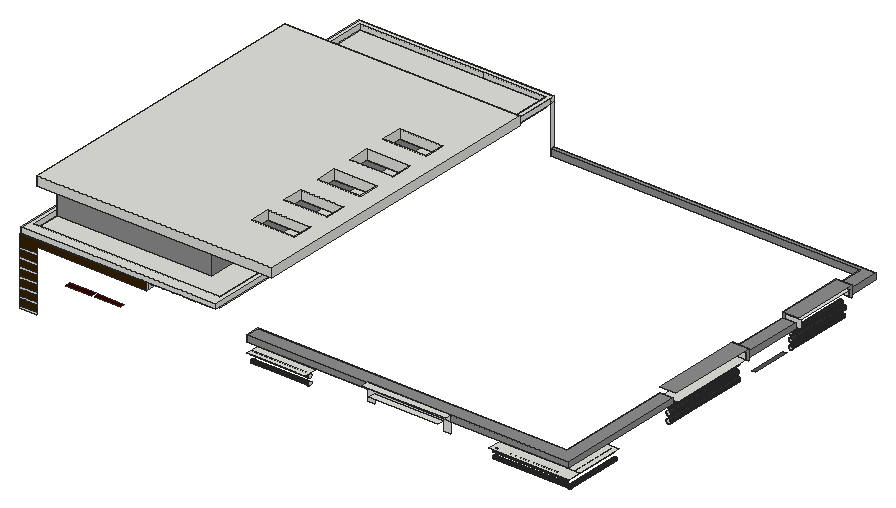
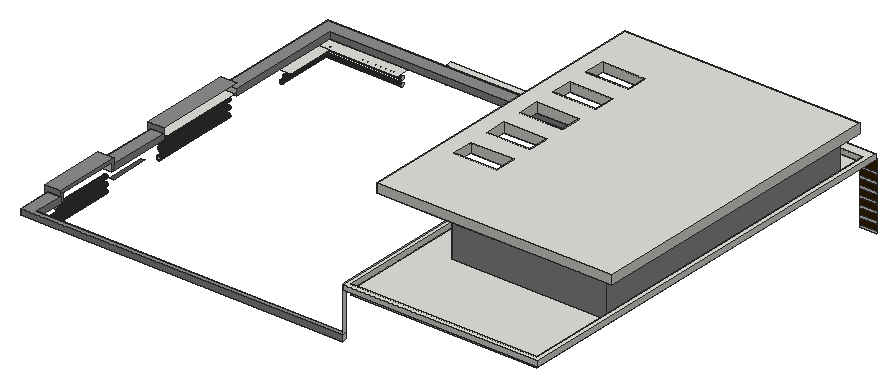
# SketchUp Ruby script. Lengths in inches.
U = 1.inch
M = Sketchup.active_model
def pt(a) = Geom::Point3d.new(a.map { |v| v * U })
def face(e, loops, mat)
  f = e.add_face(loops[0].map { |a| pt(a) })
  loops[1..].each { |l| e.add_face(l.map { |a| pt(a) }).erase! }
  f.material = f.back_material = mat if mat
  f
end
# faces: each face lists its corners as indices into pts; further lists are holes
def faces(e, pts, list, mat = nil) = list.each { |f| face(e, (f[0].is_a?(Array) ? f : [f]).map { |l| l.map { |i| pts[i] } }, mat) }
# xy, xz, yz: faces in a plane at the given z, y or x. An outline is a flat list of corners, or four numbers for a rectangle; further outlines are holes
def ring(l) = l.size == 4 ? [[l[0], l[1]], [l[2], l[1]], [l[2], l[3]], [l[0], l[3]]] : l.each_slice(2).to_a
def flat(e, list, mat, &to3) = list.each { |f| face(e, (f[0].is_a?(Array) ? f : [f]).map { |l| ring(l).map { |u, v| to3.(u, v) } }, mat) }
def xy(e, z, list, mat = nil) = flat(e, list, mat) { |x, y| [x, y, z] }
def xz(e, y, list, mat = nil) = flat(e, list, mat) { |x, z| [x, y, z] }
def yz(e, x, list, mat = nil) = flat(e, list, mat) { |y, z| [x, y, z] }
def lines(e, pts, list) = list.each { |a, b| e.add_line(pt(pts[a]), pt(pts[b])) }
# prism: a flat outline (further loops are holes) pulled along v
def prism(e, loops, v, mat = nil)
  f = face(e, loops, mat); d = Geom::Vector3d.new(v.map { |x| x * U })
  f.pushpull(f.normal.samedirection?(d) ? d.length : -d.length)
end
def box(e, o, s, mat = nil) = prism(e, [[o, [o[0] + s[0], o[1], o[2]], [o[0] + s[0], o[1] + s[1], o[2]], [o[0], o[1] + s[1], o[2]]]], [0, 0, s[2]], mat)
def at(x, y, z, deg = 0) = Geom::Transformation.translation(pt([x, y, z])) * Geom::Transformation.rotation(ORIGIN, Z_AXIS, deg.degrees)
def axes(o, x, y, z) = Geom::Transformation.new([*x, 0, *y, 0, *z, 0, *pt(o).to_a, 1])
def part(name) = M.definitions.add(name)
# library, detail: a bought-in or finely detailed component or shape, given as its bounding box
def library(name, o, s) = part(name).tap { |d| box(d.entities, o, s) }
def detail(e, o, s) = box(e.add_group.entities, o, s)
def put(e, d, t, mat = nil) = e.add_instance(d, t).tap { |i| i.material = mat if mat }
def group(e, t, mat = nil) = e.add_group.tap { |g| g.transformation = t; g.material = mat if mat }.entities
root = M.entities
M.materials.add("[Color A08]").color = [56, 34, 0]
M.materials.add("[Color A08]1").color = [63, 0, 0]
M.materials.add("[Color M04]").color = [142, 142, 142]
M.materials.add("[Color M06]").color = [86, 86, 86]
M.materials.add("[Color M07]").color = [58, 58, 58]
xy(root,396,[[746.25,843.78,750.625,894.65]],"[Color M06]")
xy(root,403.48,[[329.75,539.27,405.75,557.27],[645.89,539.27,750.625,557.27],[733.6875,557.27,750.625,621.15]])
xy(root,415.22,[[496.66,529.59,587.54,539.27]])
xy(root,417,[[329.75,539.27,750.625,557.27],[733.6875,557.27,750.625,709.18],[733.6875,828.03,750.625,909.39],[733.6875,996.8,733.6875,1035.15,329.75,1035.15,329.75,1041.15,750.625,1041.15,750.625,996.8]])
xy(root,419.97,[[733.6875,712.4,754.75,823.78]])
xy(root,424.875,[[329.75,539.27,750.625,539.27,750.625,709.18,733.6875,709.18,733.6875,557.27,329.75,557.27],[733.6875,828.03,750.625,909.39],[733.6875,996.8,750.625,996.8,750.625,1041.15,329.75,1041.15,329.75,1035.15,733.6875,1035.15]],"[Color M04]")
xy(root,425.5625,[[488.01,529.59,597.14,539.27]])
xy(root,428.02,[[733.6875,912.34,754.75,992.73]])
xy(root,430.67,[[128.05,496.71,161.69,502.71],[165.04,496.71,198.99,502.71]],"[Color A08]1")
xy(root,431.5625,[[733.6875,709.18,754.75,828.03],[733.6875,909.39,754.75,996.8]],"[Color M04]")
xy(root,468.42,[[96.69,487.84,233.4,496.71],[233.4,487.84,241.19,496.71]])
xy(root,471,[[81.5,502.71,323.75,1035.15]])
xy(root,477,[[75.5,487.84,233.4,489.27],[233.4,487.84,241.19,489.27],[241.19,489.02,247.4,489.27],[255.19,489.02,261.4,489.27],[269.19,489.02,275.4,489.27],
  [283.19,489.02,289.4,489.27],[297.19,489.02,303.4,489.27],[75.5,489.27,233.4,496.71],[233.4,489.27,241.19,496.71],[241.19,489.27,247.4,496.71],
  [247.4,489.27,255.19,496.71],[255.19,489.27,261.4,496.71],[261.4,489.27,269.19,496.71],[269.19,489.27,275.4,496.71],[275.4,489.27,283.19,496.71],
  [283.19,489.27,289.4,496.71],[289.4,489.27,297.19,496.71],[297.19,489.27,303.4,496.71],[303.4,489.27,311.19,496.71],[311.19,489.27,317.4,496.71],
  [317.4,489.27,325.19,496.71],[81.5,502.71,323.75,502.71,323.75,1035.15,81.5,1035.15,81.5,920.84,283.1875,920.84,283.1875,540.53,81.5,540.53]])
xy(root,483.8125,[[[75.5,489.27,329.75,1041.15],[81.5,502.71,323.75,1035.15]]])
xy(root,519.8125,[[73.9375,516.34,81.5,920.84],[[81.5,516.34,81.5,540.53,283.1875,540.53,283.1875,920.84,381.1875,920.84,381.1875,516.34],[303.02,580.77,358.89,608.21],[303.02,634.08,358.89,661.52],[303.02,688.46,358.89,715.89],[303.02,741.58,358.89,769.02],[303.02,795.89,358.89,823.33]],[81.5,540.53,283.1875,920.84]])
xy(root,531.8125,[[[73.9375,516.34,381.1875,920.84],[303.02,795.89,358.89,823.33],[303.02,741.58,358.89,769.02],[303.02,688.46,358.89,715.89],[303.02,634.08,358.89,661.52],[303.02,580.77,358.89,608.21]]])
xz(root,487.84,[[75.5,389.53,96.69,392.83],[75.5,401.03,96.69,404.33],[75.5,412.53,96.69,415.83],[75.5,424.03,96.69,427.33],[75.5,435.53,96.69,438.83],
  [75.5,447.03,96.69,450.33],[75.5,458.53,96.69,461.83]])
xz(root,487.84,[[75.5,392.83,96.69,401.03],[75.5,404.33,96.69,412.53],[75.5,415.83,96.69,424.03],[75.5,427.33,96.69,435.53],[75.5,438.83,96.69,447.03],
  [75.5,450.33,96.69,458.53],[75.5,461.83,96.69,461.83,96.69,468.42,241.19,468.42,241.19,477,75.5,477]],"[Color A08]")
xz(root,489.27,[[75.5,477,329.75,483.8125]])
xz(root,502.71,[[81.5,471,303.1875,477],[303.1875,471,323.75,477],[81.5,477,241.19,483.8125],[241.19,477,303.1875,483.8125],[303.1875,477,323.75,483.8125]])
xz(root,516.34,[[73.9375,519.8125,381.1875,531.8125]])
xz(root,539.27,[[488.01,403.48,488.01,417,597.14,417,597.14,403.48,587.54,403.48,587.54,415.22,496.66,415.22,496.66,403.48],[488.01,417,597.14,424.875],[488.01,424.875,597.14,425.5625]])
xz(root,539.27,[[329.75,417,488.01,424.875],[597.14,417,750.625,424.875]],"[Color M04]")
xz(root,540.53,[[81.5,477,283.1875,519.8125]],"[Color M04]")
xz(root,557.27,[[329.75,417,733.6875,424.875]],"[Color M04]")
xz(root,580.77,[[303.02,519.8125,358.89,531.8125]])
xz(root,608.21,[[303.02,519.8125,358.89,531.8125]])
xz(root,634.08,[[303.02,519.8125,358.89,531.8125]])
xz(root,661.52,[[303.02,519.8125,358.89,531.8125]])
xz(root,688.46,[[303.02,519.8125,358.89,531.8125]])
xz(root,709.18,[[733.6875,417,750.625,424.875]])
xz(root,712.4,[[742.21,389.57,742.97,389.67,743.68,389.97,744.29,390.43,744.75,391.04,745.05,391.75,745.15,392.51,745.05,393.27,744.75,393.98,744.29,394.59,743.68,395.06,742.97,395.35,742.21,395.45,741.45,395.35,740.74,395.06,740.13,394.59,739.67,393.98,739.37,393.27,739.27,392.51,739.37,391.75,739.67,391.04,740.13,390.43,740.74,389.97,741.45,389.67],[742.21,399.14,742.97,399.24,743.68,399.53,744.29,400,744.75,400.61,745.05,401.3125,745.15,402.07,745.05,402.83,744.75,403.54,744.29,404.15,743.68,404.62,742.97,404.91,742.21,405.01,741.45,404.91,740.74,404.62,740.13,404.15,739.67,403.54,739.37,402.83,739.27,402.07,739.37,401.3125,739.67,400.61,740.13,400,740.74,399.53,741.45,399.24],[742.21,408.57,742.97,408.67,743.68,408.97,744.29,409.43,744.75,410.04,745.05,410.75,745.15,411.51,745.05,412.27,744.75,412.98,744.29,413.59,743.68,414.06,742.97,414.35,742.21,414.45,741.45,414.35,740.74,414.06,740.13,413.59,739.67,412.98,739.37,412.27,739.27,411.51,739.37,410.75,739.67,410.04,740.13,409.43,740.74,408.97,741.45,408.67]])
xz(root,715.89,[[303.02,519.8125,358.89,531.8125]])
xz(root,741.58,[[303.02,519.8125,358.89,531.8125]])
xz(root,769.02,[[303.02,519.8125,358.89,531.8125]])
xz(root,795.89,[[303.02,519.8125,358.89,531.8125]])
xz(root,823.33,[[303.02,519.8125,358.89,531.8125]])
xz(root,824.97,[[742.21,408.57,741.45,408.67,740.74,408.97,740.13,409.43,739.67,410.04,739.37,410.75,739.27,411.51,739.37,412.27,739.67,412.98,740.13,413.59,740.74,414.06,741.45,414.35,742.21,414.45,742.97,414.35,743.68,414.06,744.29,413.59,744.75,412.98,745.05,412.27,745.15,411.51,745.05,410.75,744.75,410.04,744.29,409.43,743.68,408.97,742.97,408.67]])
xz(root,825.78,[[742.21,389.57,741.45,389.67,740.74,389.97,740.13,390.43,739.67,391.04,739.37,391.75,739.27,392.51,739.37,393.27,739.67,393.98,740.13,394.59,740.74,395.06,741.45,395.35,742.21,395.45,742.97,395.35,743.68,395.06,744.29,394.59,744.75,393.98,745.05,393.27,745.15,392.51,745.05,391.75,744.75,391.04,744.29,390.43,743.68,389.97,742.97,389.67]])
xz(root,828.03,[[733.6875,417,750.625,424.875]])
xz(root,828.03,[[750.625,417,750.625,424.875,733.6875,424.875,733.6875,431.5625,754.75,431.5625,754.75,417]],"[Color M04]")
xz(root,909.39,[[733.6875,417,750.625,424.875]])
xz(root,912.34,[[741.96,388.71,742.64,388.8,743.28,389.06,743.82,389.48,744.24,390.02,744.5,390.65,744.59,391.33,744.5,392.01,744.24,392.65,743.82,393.1875,743.28,393.61,742.64,393.87,741.96,393.96,741.28,393.87,740.65,393.61,740.11,393.1875,739.69,392.65,739.43,392.01,739.34,391.33,739.43,390.65,739.69,390.02,740.11,389.48,740.65,389.06,741.28,388.8],[741.96,397.33,742.64,397.42,743.28,397.68,743.82,398.1,744.24,398.65,744.5,399.28,744.59,399.96,744.5,400.64,744.24,401.27,743.82,401.8125,743.28,402.23,742.64,402.49,741.96,402.58,741.28,402.49,740.65,402.23,740.11,401.8125,739.69,401.27,739.43,400.64,739.34,399.96,739.43,399.28,739.69,398.65,740.11,398.1,740.65,397.68,741.28,397.42],[741.96,406.27,742.64,406.36,743.28,406.62,743.82,407.04,744.24,407.58,744.5,408.22,744.59,408.9,744.5,409.57,744.24,410.21,743.82,410.75,743.28,411.17,742.64,411.43,741.96,411.52,741.28,411.43,740.65,411.17,740.11,410.75,739.69,410.21,739.43,409.57,739.34,408.9,739.43,408.22,739.69,407.58,740.11,407.04,740.65,406.62,741.28,406.36],[733.6875,417,754.75,428.02]])
xz(root,920.84,[[73.9375,519.8125,381.1875,531.8125]])
xz(root,920.84,[[81.5,477,283.1875,519.8125]],"[Color M04]")
xz(root,994.41,[[741.96,406.27,741.28,406.36,740.65,406.62,740.11,407.04,739.69,407.58,739.43,408.22,739.34,408.9,739.43,409.57,739.69,410.21,740.11,410.75,740.65,411.17,741.28,411.43,741.96,411.52,742.64,411.43,743.28,411.17,743.82,410.75,744.24,410.21,744.5,409.57,744.59,408.9,744.5,408.22,744.24,407.58,743.82,407.04,743.28,406.62,742.64,406.36]])
xz(root,996.8,[[733.6875,417,750.625,424.875]])
xz(root,996.8,[[750.625,417,750.625,424.875,733.6875,424.875,733.6875,431.5625,754.75,431.5625,754.75,417]],"[Color M04]")
xz(root,997.78,[[741.96,388.71,741.28,388.8,740.65,389.06,740.11,389.48,739.69,390.02,739.43,390.65,739.34,391.33,739.43,392.01,739.69,392.65,740.11,393.1875,740.65,393.61,741.28,393.87,741.96,393.96,742.64,393.87,743.28,393.61,743.82,393.1875,744.24,392.65,744.5,392.01,744.59,391.33,744.5,390.65,744.24,390.02,743.82,389.48,743.28,389.06,742.64,388.8]])
xz(root,999.66,[[741.96,397.33,741.28,397.42,740.65,397.68,740.11,398.1,739.69,398.65,739.43,399.28,739.34,399.96,739.43,400.64,739.69,401.27,740.11,401.8125,740.65,402.23,741.28,402.49,741.96,402.58,742.64,402.49,743.28,402.23,743.82,401.8125,744.24,401.27,744.5,400.64,744.59,399.96,744.5,399.28,744.24,398.65,743.82,398.1,743.28,397.68,742.64,397.42]])
xz(root,1035.15,[[81.5,471,323.75,477],[81.5,477,241.19,483.8125],[241.19,477,323.75,483.8125]])
xz(root,1035.15,[[329.75,417,733.6875,424.875]],"[Color M04]")
xz(root,1041.15,[[75.5,477,329.75,483.8125]])
xz(root,1041.15,[[329.75,417,750.625,424.875]],"[Color M04]")
yz(root,73.9375,[[516.34,519.8125,920.84,531.8125]])
yz(root,75.5,[[489.27,477,1041.15,483.8125]])
yz(root,81.5,[[502.71,471,1035.15,471,1035.15,477,920.84,477,920.84,483.8125,540.53,483.8125,540.53,477,502.71,477],[502.71,477,540.53,483.8125],[920.84,477,1035.15,483.8125]])
yz(root,81.5,[[540.53,483.8125,920.84,519.8125]],"[Color M04]")
yz(root,241.19,[[487.84,468.42,489.02,477],[489.02,468.42,496.71,477]])
yz(root,283.1875,[[540.53,477,920.84,519.8125]],"[Color M04]")
yz(root,303.02,[[580.77,519.8125,608.21,531.8125],[634.08,519.8125,661.52,531.8125],[688.46,519.8125,715.89,531.8125],[741.58,519.8125,769.02,531.8125],[795.89,519.8125,823.33,531.8125]])
yz(root,323.75,[[502.71,471,1035.15,477],[502.71,477,1035.15,483.8125]])
yz(root,329.75,[[539.27,417,557.27,424.875],[1035.15,417,1041.15,424.875],[1035.15,424.875,1041.15,477],[489.27,477,1035.15,483.8125],[1035.15,477,1041.15,483.8125]])
yz(root,358.89,[[580.77,519.8125,608.21,531.8125],[634.08,519.8125,661.52,531.8125],[688.46,519.8125,715.89,531.8125],[741.58,519.8125,769.02,531.8125],[795.89,519.8125,823.33,531.8125]])
yz(root,381.1875,[[516.34,519.8125,920.84,531.8125]])
yz(root,405.75,[[548.47,388.74,549.02,388.81,549.53,389.02,549.97,389.36,550.3125,389.8,550.52,390.3125,550.6,390.86,550.52,391.41,550.3125,391.92,549.97,392.36,549.53,392.7,549.02,392.91,548.47,392.99,547.92,392.91,547.41,392.7,546.97,392.36,546.63,391.92,546.42,391.41,546.35,390.86,546.42,390.3125,546.63,389.8,546.97,389.36,547.41,389.02,547.92,388.81],[548.47,397.42,549.02,397.5,549.53,397.71,549.97,398.05,550.3125,398.49,550.52,399,550.6,399.55,550.52,400.1,550.3125,400.61,549.97,401.05,549.53,401.39,549.02,401.6,548.47,401.67,547.92,401.6,547.41,401.39,546.97,401.05,546.63,400.61,546.42,400.1,546.35,399.55,546.42,399,546.63,398.49,546.97,398.05,547.41,397.71,547.92,397.5]])
yz(root,645.89,[[548.01,387.84,547.45,387.91,546.92,388.13,546.47,388.48,546.12,388.93,545.9,389.46,545.83,390.02,545.9,390.59,546.12,391.12,546.47,391.57,546.92,391.92,547.45,392.14,548.01,392.21,548.58,392.14,549.11,391.92,549.5625,391.57,549.91,391.12,550.13,390.59,550.2,390.02,550.13,389.46,549.91,388.93,549.5625,388.48,549.11,388.13,548.58,387.91],[548.01,395.96,547.45,396.04,546.92,396.25,546.47,396.6,546.12,397.06,545.9,397.58,545.83,398.15,545.9,398.72,546.12,399.24,546.47,399.7,546.92,400.04,547.45,400.26,548.01,400.34,548.58,400.26,549.11,400.04,549.5625,399.7,549.91,399.24,550.13,398.72,550.2,398.15,550.13,397.58,549.91,397.06,549.5625,396.6,549.11,396.25,548.58,396.04]])
yz(root,733.6875,[[557.27,417,709.18,424.875],[828.03,417,909.39,424.875],[909.39,417,909.39,431.5625,996.8,431.5625,996.8,428.02,912.34,428.02,912.34,417],[992.73,417,996.8,428.02],[996.8,417,1035.15,424.875]],"[Color M04]")
yz(root,750.625,[[539.27,417,709.18,424.875],[828.03,417,909.39,424.875],[996.8,417,1041.15,424.875]],"[Color M04]")
p = [[645.89,547.45,387.91],[645.89,548.01,387.84],[745.76,548.01,387.84],[746.33,547.45,387.91],[745.76,621.15,387.84],[746.33,621.15,387.91],
  [645.89,548.58,387.91],[745.2,548.58,387.91],[745.2,621.15,387.91],[645.89,546.92,388.13],[746.86,546.92,388.13],[746.86,621.15,388.13],
  [645.89,549.11,388.13],[744.67,549.11,388.13],[744.67,621.15,388.13],[645.89,546.47,388.48],[747.31,546.47,388.48],[747.31,621.15,388.48],
  [645.89,549.5625,388.48],[744.22,549.5625,388.48],[744.22,621.15,388.48],[645.89,546.12,388.93],[747.66,546.12,388.93],[747.66,621.15,388.93],
  [645.89,549.91,388.93],[743.87,549.91,388.93],[743.87,621.15,388.93],[405.75,548.47,388.74],[405.75,547.92,388.81],[329.75,547.92,388.81],
  [329.75,548.47,388.74],[405.75,549.02,388.81],[329.75,549.02,388.81],[741.96,912.34,388.71],[741.28,912.34,388.8],[741.28,997.78,388.8],
  [741.96,997.78,388.71],[742.64,912.34,388.8],[742.64,997.78,388.8],[405.75,547.41,389.02],[329.75,547.41,389.02],[405.75,549.53,389.02],
  [329.75,549.53,389.02],[740.65,912.34,389.06],[740.65,997.78,389.06],[743.28,912.34,389.06],[743.28,997.78,389.06],[645.89,545.9,389.46],
  [747.875,545.9,389.46],[747.875,621.15,389.46],[645.89,550.13,389.46],[743.65,550.13,389.46],[743.65,621.15,389.46],[405.75,546.97,389.36],
  [329.75,546.97,389.36],[405.75,549.97,389.36],[329.75,549.97,389.36],[740.11,912.34,389.48],[740.11,997.78,389.48],[743.82,912.34,389.48],
  [743.82,997.78,389.48],[405.75,546.63,389.8],[329.75,546.63,389.8],[405.75,550.3125,389.8],[329.75,550.3125,389.8],[645.89,545.83,390.02],
  [747.95,545.83,390.02],[747.95,621.15,390.02],[645.89,550.2,390.02],[743.58,550.2,390.02],[743.58,621.15,390.02],[739.69,912.34,390.02],
  [739.69,997.78,390.02],[744.24,912.34,390.02],[744.24,997.78,390.02],[742.21,712.4,389.57],[741.45,712.4,389.67],[741.45,825.78,389.67],
  [742.21,825.78,389.57],[742.97,712.4,389.67],[742.97,825.78,389.67],[740.74,712.4,389.97],[740.74,825.78,389.97],[743.68,712.4,389.97],
  [743.68,825.78,389.97],[405.75,546.42,390.3125],[329.75,546.42,390.3125],[405.75,550.52,390.3125],[329.75,550.52,390.3125],[645.89,545.9,390.59],
  [747.875,545.9,390.59],[747.875,621.15,390.59],[645.89,550.13,390.59],[743.65,550.13,390.59],[743.65,621.15,390.59],[740.13,712.4,390.43],
  [740.13,825.78,390.43],[744.29,712.4,390.43],[744.29,825.78,390.43],[739.43,912.34,390.65],[739.43,997.78,390.65],[744.5,912.34,390.65],
  [744.5,997.78,390.65],[405.75,546.35,390.86],[329.75,546.35,390.86],[405.75,550.6,390.86],[329.75,550.6,390.86],[739.67,712.4,391.04],
  [739.67,825.78,391.04],[744.75,712.4,391.04],[744.75,825.78,391.04],[645.89,546.12,391.12],[747.66,546.12,391.12],[747.66,621.15,391.12],
  [645.89,549.91,391.12],[743.87,549.91,391.12],[743.87,621.15,391.12],[739.34,912.34,391.33],[739.34,997.78,391.33],[744.59,912.34,391.33],
  [744.59,997.78,391.33],[405.75,546.42,391.41],[329.75,546.42,391.41],[405.75,550.52,391.41],[329.75,550.52,391.41],[739.37,712.4,391.75],
  [739.37,825.78,391.75],[745.05,712.4,391.75],[745.05,825.78,391.75],[645.89,546.47,391.57],[747.31,546.47,391.57],[747.31,621.15,391.57],
  [645.89,549.5625,391.57],[744.22,549.5625,391.57],[744.22,621.15,391.57],[739.43,912.34,392.01],[739.43,997.78,392.01],[744.5,912.34,392.01],
  [744.5,997.78,392.01],[405.75,546.63,391.92],[329.75,546.63,391.92],[405.75,550.3125,391.92],[329.75,550.3125,391.92],[645.89,546.92,391.92],
  [746.86,546.92,391.92],[746.86,621.15,391.92],[645.89,549.11,391.92],[744.67,549.11,391.92],[744.67,621.15,391.92],[739.27,712.4,392.51],
  [739.27,825.78,392.51],[745.15,712.4,392.51],[745.15,825.78,392.51],[405.75,546.97,392.36],[329.75,546.97,392.36],[645.89,547.45,392.14],
  [746.33,547.45,392.14],[746.33,621.15,392.14],[645.89,548.58,392.14],[745.2,548.58,392.14],[745.2,621.15,392.14],[405.75,549.97,392.36],
  [329.75,549.97,392.36],[739.69,912.34,392.65],[739.69,997.78,392.65],[744.24,912.34,392.65],[744.24,997.78,392.65],[645.89,548.01,392.21],
  [745.76,548.01,392.21],[745.76,621.15,392.21],[405.75,547.41,392.7],[329.75,547.41,392.7],[405.75,549.53,392.7],[329.75,549.53,392.7],
  [739.37,712.4,393.27],[739.37,825.78,393.27],[745.05,712.4,393.27],[745.05,825.78,393.27],[740.11,912.34,393.1875],[740.11,997.78,393.1875],
  [743.82,912.34,393.1875],[743.82,997.78,393.1875],[405.75,547.92,392.91],[329.75,547.92,392.91],[405.75,549.02,392.91],[329.75,549.02,392.91],
  [405.75,548.47,392.99],[329.75,548.47,392.99],[740.65,912.34,393.61],[740.65,997.78,393.61],[743.28,912.34,393.61],[743.28,997.78,393.61],
  [739.67,712.4,393.98],[739.67,825.78,393.98],[744.75,712.4,393.98],[744.75,825.78,393.98],[741.28,912.34,393.87],[741.28,997.78,393.87],
  [742.64,912.34,393.87],[742.64,997.78,393.87],[741.96,912.34,393.96],[741.96,997.78,393.96],[740.13,712.4,394.59],[740.13,825.78,394.59],
  [744.29,712.4,394.59],[744.29,825.78,394.59],[740.74,712.4,395.06],[740.74,825.78,395.06],[743.68,712.4,395.06],[743.68,825.78,395.06],
  [741.45,712.4,395.35],[741.45,825.78,395.35],[742.97,712.4,395.35],[742.97,825.78,395.35],[742.21,712.4,395.45],[742.21,825.78,395.45],
  [645.89,546.92,396.25],[645.89,547.45,396.04],[742.45,547.45,396.04],[742.98,546.92,396.25],[742.45,621.15,396.04],[742.98,621.15,396.25],
  [645.89,548.01,395.96],[741.89,548.01,395.96],[741.89,621.15,395.96],[645.89,548.58,396.04],[741.32,548.58,396.04],[741.32,621.15,396.04],
  [645.89,549.11,396.25],[740.79,549.11,396.25],[740.79,621.15,396.25],[645.89,546.47,396.6],[743.44,546.47,396.6],[743.44,621.15,396.6],
  [645.89,549.5625,396.6],[740.34,549.5625,396.6],[740.34,621.15,396.6],[645.89,546.12,397.06],[743.78,546.12,397.06],[743.78,621.15,397.06],
  [645.89,549.91,397.06],[739.99,549.91,397.06],[739.99,621.15,397.06],[645.89,545.9,397.58],[744,545.9,397.58],[744,621.15,397.58],
  [645.89,550.13,397.58],[739.78,550.13,397.58],[739.78,621.15,397.58],[741.96,912.34,397.33],[741.28,912.34,397.42],[741.28,999.66,397.42],
  [741.96,999.66,397.33],[742.64,912.34,397.42],[742.64,999.66,397.42],[405.75,548.47,397.42],[405.75,547.92,397.5],[329.75,547.92,397.5],
  [329.75,548.47,397.42],[405.75,549.02,397.5],[329.75,549.02,397.5],[740.65,912.34,397.68],[740.65,999.66,397.68],[743.28,912.34,397.68],
  [743.28,999.66,397.68],[405.75,547.41,397.71],[329.75,547.41,397.71],[405.75,549.53,397.71],[329.75,549.53,397.71],[645.89,545.83,398.15],
  [744.08,545.83,398.15],[744.08,621.15,398.15],[645.89,550.2,398.15],[739.7,550.2,398.15],[739.7,621.15,398.15],[405.75,546.97,398.05],
  [329.75,546.97,398.05],[405.75,549.97,398.05],[329.75,549.97,398.05],[740.11,912.34,398.1],[740.11,999.66,398.1],[743.82,912.34,398.1],
  [743.82,999.66,398.1],[405.75,546.63,398.49],[329.75,546.63,398.49],[405.75,550.3125,398.49],[329.75,550.3125,398.49],[645.89,545.9,398.72],
  [744,545.9,398.72],[744,621.15,398.72],[645.89,550.13,398.72],[739.78,550.13,398.72],[739.78,621.15,398.72],[739.69,912.34,398.65],
  [739.69,999.66,398.65],[744.24,912.34,398.65],[744.24,999.66,398.65],[405.75,546.42,399],[329.75,546.42,399],[405.75,550.52,399],
  [329.75,550.52,399],[739.43,912.34,399.28],[739.43,999.66,399.28],[744.5,912.34,399.28],[744.5,999.66,399.28],[645.89,546.12,399.24],
  [743.78,546.12,399.24],[743.78,621.15,399.24],[645.89,549.91,399.24],[739.99,549.91,399.24],[739.99,621.15,399.24],[405.75,546.35,399.55],
  [329.75,546.35,399.55],[405.75,550.6,399.55],[329.75,550.6,399.55],[742.21,712.4,399.14],[741.45,712.4,399.24],[741.45,823.78,399.24],
  [742.21,823.78,399.14],[742.97,712.4,399.24],[742.97,823.78,399.24],[645.89,546.47,399.7],[743.44,546.47,399.7],[743.44,621.15,399.7],
  [645.89,549.5625,399.7],[740.34,549.5625,399.7],[740.34,621.15,399.7],[740.74,712.4,399.53],[740.74,823.78,399.53],[743.68,712.4,399.53],
  [743.68,823.78,399.53],[739.34,912.34,399.96],[739.34,999.66,399.96],[744.59,912.34,399.96],[744.59,999.66,399.96],[405.75,546.42,400.1],
  [329.75,546.42,400.1],[405.75,550.52,400.1],[329.75,550.52,400.1],[740.13,712.4,400],[740.13,823.78,400],[744.29,712.4,400],
  [744.29,823.78,400],[645.89,546.92,400.04],[742.98,546.92,400.04],[742.98,621.15,400.04],[645.89,549.11,400.04],[740.79,549.11,400.04],
  [740.79,621.15,400.04],[645.89,547.45,400.26],[742.45,547.45,400.26],[742.45,621.15,400.26],[645.89,548.58,400.26],[741.32,548.58,400.26],
  [741.32,621.15,400.26],[739.67,712.4,400.61],[739.67,823.78,400.61],[744.75,712.4,400.61],[744.75,823.78,400.61],[739.43,912.34,400.64],
  [739.43,999.66,400.64],[744.5,912.34,400.64],[744.5,999.66,400.64],[405.75,546.63,400.61],[329.75,546.63,400.61],[405.75,550.3125,400.61],
  [329.75,550.3125,400.61],[645.89,548.01,400.34],[741.89,548.01,400.34],[741.89,621.15,400.34],[405.75,546.97,401.05],[329.75,546.97,401.05],
  [405.75,549.97,401.05],[329.75,549.97,401.05],[739.37,712.4,401.3125],[739.37,823.78,401.3125],[745.05,712.4,401.3125],[745.05,823.78,401.3125],
  [739.69,912.34,401.27],[739.69,999.66,401.27],[744.24,912.34,401.27],[744.24,999.66,401.27],[405.75,547.41,401.39],[329.75,547.41,401.39],
  [405.75,549.53,401.39],[329.75,549.53,401.39],[739.27,712.4,402.07],[739.27,823.78,402.07],[745.15,712.4,402.07],[745.15,823.78,402.07],
  [740.11,912.34,401.8125],[740.11,999.66,401.8125],[743.82,912.34,401.8125],[743.82,999.66,401.8125],[405.75,547.92,401.6],[329.75,547.92,401.6],
  [405.75,549.02,401.6],[329.75,549.02,401.6],[405.75,548.47,401.67],[329.75,548.47,401.67],[740.65,912.34,402.23],[740.65,999.66,402.23],
  [743.28,912.34,402.23],[743.28,999.66,402.23],[739.37,712.4,402.83],[739.37,823.78,402.83],[745.05,712.4,402.83],[745.05,823.78,402.83],
  [741.28,912.34,402.49],[741.28,999.66,402.49],[742.64,912.34,402.49],[742.64,999.66,402.49],[741.96,912.34,402.58],[741.96,999.66,402.58],
  [739.67,712.4,403.54],[739.67,823.78,403.54],[744.75,712.4,403.54],[744.75,823.78,403.54],[740.13,712.4,404.15],[740.13,823.78,404.15],
  [744.29,712.4,404.15],[744.29,823.78,404.15],[740.74,712.4,404.62],[740.74,823.78,404.62],[743.68,712.4,404.62],[743.68,823.78,404.62],
  [741.45,712.4,404.91],[741.45,823.78,404.91],[742.97,712.4,404.91],[742.97,823.78,404.91],[742.21,712.4,405.01],[742.21,823.78,405.01],
  [741.96,912.34,406.27],[741.28,912.34,406.36],[741.28,994.41,406.36],[741.96,994.41,406.27],[742.64,912.34,406.36],[742.64,994.41,406.36],
  [740.65,912.34,406.62],[740.65,994.41,406.62],[743.28,912.34,406.62],[743.28,994.41,406.62],[740.11,912.34,407.04],[740.11,994.41,407.04],
  [743.82,912.34,407.04],[743.82,994.41,407.04],[739.69,912.34,407.58],[739.69,994.41,407.58],[744.24,912.34,407.58],[744.24,994.41,407.58],
  [739.43,912.34,408.22],[739.43,994.41,408.22],[744.5,912.34,408.22],[744.5,994.41,408.22],[739.34,912.34,408.9],[739.34,994.41,408.9],
  [744.59,912.34,408.9],[744.59,994.41,408.9],[742.21,712.4,408.57],[741.45,712.4,408.67],[741.45,824.97,408.67],[742.21,824.97,408.57],
  [742.97,712.4,408.67],[742.97,824.97,408.67],[740.74,712.4,408.97],[740.74,824.97,408.97],[743.68,712.4,408.97],[743.68,824.97,408.97],
  [739.43,912.34,409.57],[739.43,994.41,409.57],[744.5,912.34,409.57],[744.5,994.41,409.57],[740.13,712.4,409.43],[740.13,824.97,409.43],
  [744.29,712.4,409.43],[744.29,824.97,409.43],[739.67,712.4,410.04],[739.67,824.97,410.04],[744.75,712.4,410.04],[744.75,824.97,410.04],
  [739.69,912.34,410.21],[739.69,994.41,410.21],[744.24,912.34,410.21],[744.24,994.41,410.21],[739.37,712.4,410.75],[739.37,824.97,410.75],
  [745.05,712.4,410.75],[745.05,824.97,410.75],[740.11,912.34,410.75],[740.11,994.41,410.75],[743.82,912.34,410.75],[743.82,994.41,410.75],
  [739.27,712.4,411.51],[739.27,824.97,411.51],[745.15,712.4,411.51],[745.15,824.97,411.51],[740.65,912.34,411.17],[740.65,994.41,411.17],
  [743.28,912.34,411.17],[743.28,994.41,411.17],[741.28,912.34,411.43],[741.28,994.41,411.43],[742.64,912.34,411.43],[742.64,994.41,411.43],
  [741.96,912.34,411.52],[741.96,994.41,411.52],[739.37,712.4,412.27],[739.37,824.97,412.27],[745.05,712.4,412.27],[745.05,824.97,412.27],
  [739.67,712.4,412.98],[739.67,824.97,412.98],[744.75,712.4,412.98],[744.75,824.97,412.98],[740.13,712.4,413.59],[740.13,824.97,413.59],
  [744.29,712.4,413.59],[744.29,824.97,413.59],[740.74,712.4,414.06],[740.74,824.97,414.06],[743.68,712.4,414.06],[743.68,824.97,414.06],
  [741.45,712.4,414.35],[741.45,824.97,414.35],[742.97,712.4,414.35],[742.97,824.97,414.35],[742.21,712.4,414.45],[742.21,824.97,414.45],
  [645.89,548.01,390.02],[745.76,548.01,390.02],[745.76,621.15,390.02],[645.89,548.01,398.15],[741.89,548.01,398.15],[741.89,621.15,398.15],
  [733.6875,825.95,426.54],[731.5,825.95,426.54],[241.19,1035.15,477],[241.19,1041.15,477]]
faces(root,p,[[0,1,2,3],[3,2,4,5],[1,6,7,2],[2,7,8,4],[9,0,3,10],[10,3,5,11],[6,12,13,7],[7,13,14,8],
  [15,9,10,16],[16,10,11,17],[12,18,19,13],[13,19,20,14],[21,15,16,22],[22,16,17,23],[18,24,25,19],[19,25,26,20],
  [27,28,29,30],[31,27,30,32],[28,39,40,29],[41,31,32,42],[47,21,22,48],[48,22,23,49],[24,50,51,25],[25,51,52,26],
  [39,53,54,40],[55,41,42,56],[53,61,62,54],[63,55,56,64],[65,47,48,66],[66,48,49,67],[50,68,69,51],[51,69,70,52],
  [61,85,86,62],[87,63,64,88],[89,65,66,90],[90,66,67,91],[68,92,93,69],[69,93,94,70],[85,103,104,86],[105,87,88,106],
  [111,89,90,112],[112,90,91,113],[92,114,115,93],[93,115,116,94],[103,121,122,104],[123,105,106,124],[129,111,112,130],[130,112,113,131],
  [114,132,133,115],[115,133,134,116],[121,139,140,122],[141,123,124,142],[143,129,130,144],[144,130,131,145],[132,146,147,133],[133,147,148,134],
  [139,153,154,140],[155,143,144,156],[156,144,145,157],[146,158,159,147],[147,159,160,148],[161,141,142,162],[167,155,156,168],[168,156,157,169],
  [158,167,168,159],[159,168,169,160],[153,170,171,154],[172,161,162,173],[170,182,183,171],[184,172,173,185],[182,186,187,183],[186,184,185,187],
  [216,217,218,219],[219,218,220,221],[217,222,223,218],[218,223,224,220],[222,225,226,223],[223,226,227,224],[225,228,229,226],[226,229,230,227],
  [231,216,219,232],[232,219,221,233],[228,234,235,229],[229,235,236,230],[237,231,232,238],[238,232,233,239],[234,240,241,235],[235,241,242,236],
  [243,237,238,244],[244,238,239,245],[240,246,247,241],[241,247,248,242],[255,256,257,258],[259,255,258,260],[256,265,266,257],[267,259,260,268],
  [269,243,244,270],[270,244,245,271],[246,272,273,247],[247,273,274,248],[265,275,276,266],[277,267,268,278],[275,283,284,276],[285,277,278,286],
  [287,269,270,288],[288,270,271,289],[272,290,291,273],[273,291,292,274],[283,297,298,284],[299,285,286,300],[305,287,288,306],[306,288,289,307],
  [290,308,309,291],[291,309,310,292],[297,311,312,298],[313,299,300,314],[321,305,306,322],[322,306,307,323],[308,324,325,309],[309,325,326,310],
  [311,335,336,312],[337,313,314,338],[343,321,322,344],[344,322,323,345],[324,346,347,325],[325,347,348,326],[349,343,344,350],[350,344,345,351],
  [346,352,353,347],[347,353,354,348],[335,363,364,336],[365,337,338,366],[367,349,350,368],[368,350,351,369],[352,367,368,353],[353,368,369,354],
  [363,370,371,364],[372,365,366,373],[370,382,383,371],[384,372,373,385],[382,394,395,383],[396,384,385,397],[394,398,399,395],[398,396,397,399]],"[Color A08]")
faces(root,p,[[33,34,35,36],[37,33,36,38],[34,43,44,35],[45,37,38,46],[43,57,58,44],[59,45,46,60],[57,71,72,58],[73,59,60,74],
  [75,76,77,78],[79,75,78,80],[76,81,82,77],[83,79,80,84],[81,95,96,82],[97,83,84,98],[71,99,100,72],[101,73,74,102],
  [95,107,108,96],[109,97,98,110],[99,117,118,100],[119,101,102,120],[107,125,126,108],[127,109,110,128],[117,135,136,118],[137,119,120,138],
  [125,149,150,126],[151,127,128,152],[135,163,164,136],[165,137,138,166],[149,174,175,150],[176,151,152,177],[163,178,179,164],[180,165,166,181],
  [178,188,189,179],[190,180,181,191],[174,192,193,175],[194,176,177,195],[188,196,197,189],[198,190,191,199],[196,200,201,197],[200,198,199,201],
  [192,202,203,193],[204,194,195,205],[202,206,207,203],[208,204,205,209],[206,210,211,207],[212,208,209,213],[210,214,215,211],[214,212,213,215],
  [249,250,251,252],[253,249,252,254],[250,261,262,251],[263,253,254,264],[261,279,280,262],[281,263,264,282],[279,293,294,280],[295,281,282,296],
  [293,301,302,294],[303,295,296,304],[315,316,317,318],[319,315,318,320],[316,327,328,317],[329,319,320,330],[301,331,332,302],[333,303,304,334],
  [327,339,340,328],[341,329,330,342],[339,355,356,340],[357,341,342,358],[331,359,360,332],[361,333,334,362],[355,374,375,356],[376,357,358,377],
  [359,378,379,360],[380,361,362,381],[374,386,387,375],[388,376,377,389],[378,390,391,379],[392,380,381,393],[390,400,401,391],[402,392,393,403],
  [386,404,405,387],[406,388,389,407],[400,408,409,401],[410,402,403,411],[408,412,413,409],[412,410,411,413],[404,414,415,405],[416,406,407,417],
  [414,418,419,415],[420,416,417,421],[418,422,423,419],[424,420,421,425],[422,426,427,423],[428,424,425,429],[426,430,431,427],[430,428,429,431],
  [432,433,434,435],[436,432,435,437],[433,438,439,434],[440,436,437,441],[438,442,443,439],[444,440,441,445],[442,446,447,443],[448,444,445,449],
  [446,450,451,447],[452,448,449,453],[450,454,455,451],[456,452,453,457],[458,459,460,461],[462,458,461,463],[459,464,465,460],[466,462,463,467],
  [454,468,469,455],[470,456,457,471],[464,472,473,465],[474,466,467,475],[472,476,477,473],[478,474,475,479],[468,480,481,469],[482,470,471,483],
  [476,484,485,477],[486,478,479,487],[480,488,489,481],[490,482,483,491],[484,492,493,485],[494,486,487,495],[488,496,497,489],[498,490,491,499],
  [496,500,501,497],[502,498,499,503],[500,504,505,501],[504,502,503,505],[492,506,507,493],[508,494,495,509],[506,510,511,507],[512,508,509,513],
  [510,514,515,511],[516,512,513,517],[514,518,519,515],[520,516,517,521],[518,522,523,519],[524,520,521,525],[522,526,527,523],[526,524,525,527]],"[Color M07]")
lines(root,p,[[528,529],[529,530],[531,532],[532,533],[534,535],[536,537]])
